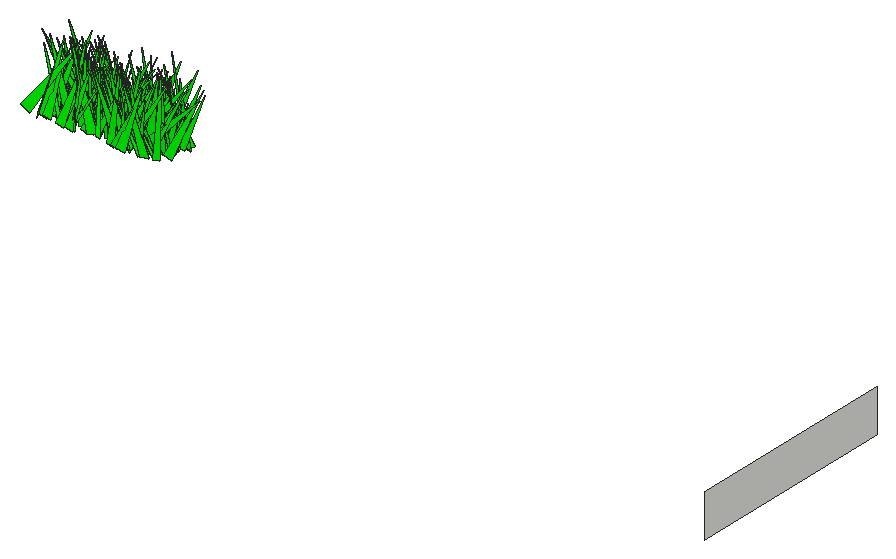
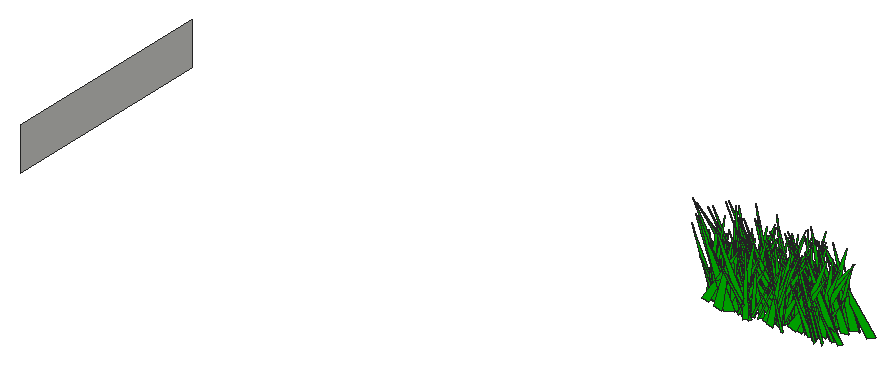
# SketchUp Ruby script. Lengths in inches.
U = 1.inch
M = Sketchup.active_model
def pt(a) = Geom::Point3d.new(a.map { |v| v * U })
def face(e, loops, mat)
  f = e.add_face(loops[0].map { |a| pt(a) })
  loops[1..].each { |l| e.add_face(l.map { |a| pt(a) }).erase! }
  f.material = f.back_material = mat if mat
  f
end
# faces: each face lists its corners as indices into pts; further lists are holes
def faces(e, pts, list, mat = nil) = list.each { |f| face(e, (f[0].is_a?(Array) ? f : [f]).map { |l| l.map { |i| pts[i] } }, mat) }
# xy, xz, yz: faces in a plane at the given z, y or x. An outline is a flat list of corners, or four numbers for a rectangle; further outlines are holes
def ring(l) = l.size == 4 ? [[l[0], l[1]], [l[2], l[1]], [l[2], l[3]], [l[0], l[3]]] : l.each_slice(2).to_a
def flat(e, list, mat, &to3) = list.each { |f| face(e, (f[0].is_a?(Array) ? f : [f]).map { |l| ring(l).map { |u, v| to3.(u, v) } }, mat) }
def xy(e, z, list, mat = nil) = flat(e, list, mat) { |x, y| [x, y, z] }
def xz(e, y, list, mat = nil) = flat(e, list, mat) { |x, z| [x, y, z] }
def yz(e, x, list, mat = nil) = flat(e, list, mat) { |y, z| [x, y, z] }
def lines(e, pts, list) = list.each { |a, b| e.add_line(pt(pts[a]), pt(pts[b])) }
# prism: a flat outline (further loops are holes) pulled along v
def prism(e, loops, v, mat = nil)
  f = face(e, loops, mat); d = Geom::Vector3d.new(v.map { |x| x * U })
  f.pushpull(f.normal.samedirection?(d) ? d.length : -d.length)
end
def box(e, o, s, mat = nil) = prism(e, [[o, [o[0] + s[0], o[1], o[2]], [o[0] + s[0], o[1] + s[1], o[2]], [o[0], o[1] + s[1], o[2]]]], [0, 0, s[2]], mat)
def at(x, y, z, deg = 0) = Geom::Transformation.translation(pt([x, y, z])) * Geom::Transformation.rotation(ORIGIN, Z_AXIS, deg.degrees)
def axes(o, x, y, z) = Geom::Transformation.new([*x, 0, *y, 0, *z, 0, *pt(o).to_a, 1])
def part(name) = M.definitions.add(name)
# library, detail: a bought-in or finely detailed component or shape, given as its bounding box
def library(name, o, s) = part(name).tap { |d| box(d.entities, o, s) }
def detail(e, o, s) = box(e.add_group.entities, o, s)
def put(e, d, t, mat = nil) = e.add_instance(d, t).tap { |i| i.material = mat if mat }
def group(e, t, mat = nil) = e.add_group.tap { |g| g.transformation = t; g.material = mat if mat }.entities
root = M.entities
M.materials.add("[0065_Lime]").color = [0, 255, 0]
c1 = part("fur_instance\#9")
p = [[0.8125,0,1.79],[0.67,-0.02,1.48],[0,-0.11,0],[0,0.11,0]]
faces(c1.entities,p,[[0,1,2,3]])
yz(root,282.96,[[0,-11.8125,39.75,-3.9375]])
put(root,c1,axes([141.5625,19.58,1.48],[2.20654,1.20218,2.33914],[-8.01635,0.06988,3.7999],[4.14751,-0.50452,6.10002]),"[0065_Lime]")
put(root,c1,axes([147.93,19.65,1.48],[-6.97873,0.43873,0.69681],[-2.96337,-0.98079,1.05602],[1.30411,0.11912,6.1285]),"[0065_Lime]")
put(root,c1,axes([144.33,18.92,1.48],[7.25336,-0.09629,0.71181],[0.1838,0.90456,2.86128],[-1.09619,-0.48551,5.18975]),"[0065_Lime]")
put(root,c1,axes([143.88,23.88,1.48],[1.3632,-0.63069,1.12453],[4.15726,0.06795,-2.05747],[2.18484,0.26422,3.21328]),"[0065_Lime]")
put(root,c1,axes([144.875,19.43,1.48],[-3.49359,1.08943,2.25762],[-7.42243,-0.60007,2.10352],[3.56638,-0.18169,6.58944]),"[0065_Lime]")
put(root,c1,axes([150.37,22.14,1.48],[-2.75165,-1.05841,0.96268],[7.17807,-0.29998,2.52342],[-2.57099,0.29525,6.01494]),"[0065_Lime]")
put(root,c1,axes([145.71,19.36,1.48],[-0.65738,0.93907,0.42813],[-6.48617,-0.10788,1.33939],[1.6937,-0.04864,5.29548]),"[0065_Lime]")
put(root,c1,axes([148.99,20.83,1.48],[-4.18903,-0.24167,0.3067],[1.732,-0.54103,1.36687],[-0.31652,0.23788,3.4204]),"[0065_Lime]")
put(root,c1,axes([145.5,20.31,1.48],[7.3444,0.3612,0.82059],[-2.31076,1.02444,-1.4263],[-1.5118,0.18888,6.16656]),"[0065_Lime]")
put(root,c1,axes([147.78,23.43,1.48],[3.54324,-1.13333,0.24164],[7.72696,0.48952,1.96765],[-2.33086,-0.10005,6.89022]),"[0065_Lime]")
put(root,c1,axes([147.25,20.59,1.48],[4.55951,-0.27108,1.43916],[1.50494,0.68003,1.13749],[-2.14174,-0.09925,3.86308]),"[0065_Lime]")
put(root,c1,axes([149.5,23.12,1.48],[-2.25393,-1.02556,0.82554],[7.20883,-0.276,1.53316],[-1.52654,0.21089,6.02119]),"[0065_Lime]")
put(root,c1,axes([147.41,21.64,1.48],[-3.74761,0.46815,0.23905],[-2.94612,-0.49143,1.69066],[1.58322,0.19368,3.71191]),"[0065_Lime]")
put(root,c1,axes([146.61,20.24,1.48],[-2.35602,0.71684,1.55449],[-5.12228,-0.39111,0.90693],[1.85452,-0.16956,4.47986]),"[0065_Lime]")
put(root,c1,axes([146.07,25.37,1.48],[6.49206,0.06434,1.15893],[-0.05568,0.90105,-1.46982],[-1.49551,0.24575,5.08571]),"[0065_Lime]")
put(root,c1,axes([144.83,23.57,1.48],[3.73059,0.98054,1.41858],[-7.08226,0.45258,1.8405],[1.25541,-0.36059,6.1675]),"[0065_Lime]")
put(root,c1,axes([145,23.73,1.48],[2.36799,1.27418,0.18786],[-8.9088,0.32039,1.48209],[1.70623,-0.09551,7.47774]),"[0065_Lime]")
put(root,c1,axes([152.77,21.72,1.48],[-6.46009,0.95745,0.30947],[-6.30621,-0.80939,-3.18772],[-2.6084,-0.41445,6.94037]),"[0065_Lime]")
put(root,c1,axes([149.78,19.83,1.48],[-2.56954,1.1411,1.85865],[-8.37179,-0.30358,-1.41229],[-1.03904,-0.3759,6.78277]),"[0065_Lime]")
put(root,c1,axes([145.34,23.82,1.48],[6.35731,-0.22767,0.53306],[1.74475,0.84708,-1.6442],[-0.10245,0.29824,5.07681]),"[0065_Lime]")
put(root,c1,axes([145.48,20.91,1.48],[5.10197,0.98969,1.68963],[-7.32568,0.66151,1.65177],[0.5059,-0.40195,6.87867]),"[0065_Lime]")
put(root,c1,axes([148.52,22.64,1.48],[-4.37999,-0.37273,0.87769],[2.35536,-0.6265,-1.13841],[1.62873,-0.09636,4.00656]),"[0065_Lime]")
put(root,c1,axes([148.85,24.07,1.48],[-4.93438,-0.47308,0.40197],[3.03876,-0.66768,-1.65014],[1.53121,-0.19947,4.57013]),"[0065_Lime]")
put(root,c1,axes([147.08,22.4,1.48],[6.97665,0.36677,2.16628],[-3.21314,0.99415,1.20661],[-1.89239,-0.33583,5.93769]),"[0065_Lime]")
put(root,c1,axes([147.11,25.87,1.48],[5.53718,0.0797,0.9196],[-0.81995,0.76935,1.03237],[-0.96306,-0.1968,4.40831]),"[0065_Lime]")
put(root,c1,axes([150.49,21.42,1.48],[-4.93557,-0.23453,0.41154],[1.74339,-0.66937,1.05115],[0.04838,0.19489,4.10557]),"[0065_Lime]")
put(root,c1,axes([151.4,24.46,1.48],[-5.52806,-1.01005,1.40888],[7.36884,-0.72767,1.64938],[-0.60725,0.36488,7.18923]),"[0065_Lime]")
put(root,c1,axes([148.9,23.33,1.48],[-4.95765,-0.84883,1.39379],[5.90771,-0.7345,-1.08569],[2.12734,0.06158,6.26314]),"[0065_Lime]")
put(root,c1,axes([147.18,22.61,1.48],[5.87849,0.29778,0.30468],[-1.98317,0.80905,-1.17995],[-0.83558,0.17474,4.944]),"[0065_Lime]")
put(root,c1,axes([148.66,22.27,1.48],[-3.00842,-0.53467,0.10404],[3.43756,-0.39133,-1.62121],[1.63632,-0.16091,3.59711]),"[0065_Lime]")
put(root,c1,axes([151.14,21.84,1.48],[-3.35195,0.85295,0.90617],[-6.1043,-0.43203,-1.31319],[-0.90765,-0.24434,5.48523]),"[0065_Lime]")
put(root,c1,axes([152.37,24.53,1.48],[-3.97671,0.93782,0.27867],[-6.39186,-0.51742,-2.00237],[-1.95047,-0.21646,5.99377]),"[0065_Lime]")
put(root,c1,axes([151.22,23.7,1.48],[-1.49671,0.82532,1.20922],[-5.79693,-0.13252,-1.71648],[-1.76135,-0.26515,4.62172]),"[0065_Lime]")
put(root,c1,axes([147.38,23.35,1.48],[1.15932,-0.85561,0.4723],[5.95948,0.1393,-1.22246],[1.37745,0.11743,4.89139]),"[0065_Lime]")
put(root,c1,axes([147.58,20.61,1.48],[1.71149,0.52944,0.12124],[-3.59338,0.22204,1.07239],[1.14269,-0.09474,3.19072]),"[0065_Lime]")
put(root,c1,axes([150.46,22.47,1.48],[1.53529,0.56905,0.27796],[-3.6294,0.21508,-1.49067],[-1.82868,0.05089,3.19191]),"[0065_Lime]")
put(root,c1,axes([149.52,23.63,1.48],[-4.03165,0.0597,1.8592],[-1.0991,-0.6155,-0.91462],[2.04862,-0.21273,3.16818]),"[0065_Lime]")
put(root,c1,axes([149.93,22.65,1.48],[-5.98029,-0.8429,0.18918],[5.44661,-0.78127,-2.72487],[2.52406,-0.31121,6.32814]),"[0065_Lime]")
put(root,c1,axes([147.69,25.28,1.48],[8.61099,-0.37367,0.75747],[2.45007,1.20083,1.42172],[-1.39136,-0.19804,7.19149]),"[0065_Lime]")
put(root,c1,axes([148.4375,24.65,1.48],[-0.04705,-1.17072,0.26335],[8.10686,-0.01706,-1.58237],[1.94856,0.04269,6.58971]),"[0065_Lime]")
put(root,c1,axes([149.85,22.76,1.48],[-6.12929,-0.74533,0.16535],[4.24135,-0.71392,-3.81017],[3.19162,-0.48262,5.38089]),"[0065_Lime]")
put(root,c1,axes([153.17,24.05,1.48],[-3.64838,-0.56917,0.80639],[3.93076,-0.40758,2.12677],[-1.39242,0.34074,3.89092]),"[0065_Lime]")
put(root,c1,axes([152.62,23.41,1.48],[-1.12028,1.15408,0.64786],[-8.03924,-0.12719,-1.60528],[-1.85986,-0.14535,6.54857]),"[0065_Lime]")
put(root,c1,axes([148.71,24.83,1.48],[2.84326,0.64249,0.39365],[-4.54228,0.38012,0.91821],[0.71259,-0.14057,4.28228]),"[0065_Lime]")
put(root,c1,axes([148.64,18.74,1.48],[2.22567,0.92219,0.99487],[-6.58515,0.27352,1.25154],[1.09663,-0.22921,5.49624]),"[0065_Lime]")
put(root,c1,axes([151.48,21.18,1.48],[-8.34339,-0.0857,2.24479],[-0.02277,-1.20659,-1.59957],[2.82621,-0.26272,6.61406]),"[0065_Lime]")
put(root,c1,axes([149.93,24.47,1.48],[4.72063,0.10631,0.85352],[-0.3936,0.64949,-1.27031],[-1.23225,0.19979,3.67549]),"[0065_Lime]")
put(root,c1,axes([151.53,23.91,1.48],[-4.16121,-0.53442,0.1089],[3.60478,-0.56246,-1.35649],[1.21978,-0.1609,4.38028]),"[0065_Lime]")
put(root,c1,axes([153.41,20.67,1.48],[3.38639,-0.8607,4.01971],[6.71512,0.71024,1.35296],[-4.10446,0.45187,5.52997]),"[0065_Lime]")
put(root,c1,axes([149.8,19.63,1.48],[8.32669,-0.46304,2.49552],[3.88184,1.1975,-1.12428],[-2.28087,0.34763,7.19685]),"[0065_Lime]")
put(root,c1,axes([152.74,20.86,1.48],[-7.78088,-0.56548,0.89942],[3.74968,-1.09155,-1.53398],[1.83234,-0.16754,6.9584]),"[0065_Lime]")
put(root,c1,axes([151.46,18.67,1.48],[7.41008,0.10379,2.59282],[0.16748,1.09537,-1.78601],[-3.26775,0.2915,5.78804]),"[0065_Lime]")
put(root,c1,axes([151.44,20.45,1.48],[5.13469,0.907,1.4446],[-6.32228,0.7604,-1.12939],[-2.20133,-0.06827,6.61322]),"[0065_Lime]")
put(root,c1,axes([147.3,20.35,1.48],[7.19198,-0.75486,0.91121],[5.17085,0.84533,-3.53719],[1.83736,0.57576,6.38791]),"[0065_Lime]")
put(root,c1,axes([153.84,19.66,1.48],[4.02373,-1.03653,3.45136],[7.56263,0.73794,1.59281],[-3.90173,0.3614,6.64659]),"[0065_Lime]")
put(root,c1,axes([151.38,24.125,1.48],[-2.16031,-0.73135,0.90472],[5.04667,-0.33506,-1.10284],[1.69026,0.06566,4.44911]),"[0065_Lime]")
put(root,c1,axes([150.92,19.02,1.48],[7.24147,-0.41945,0.98876],[2.5105,0.9975,2.01423],[-2.0212,-0.26379,6.04433]),"[0065_Lime]")
put(root,c1,axes([148.58,20.76,1.48],[9.08947,-0.29649,0.75138],[2.29764,1.20426,-2.46681],[-0.16186,0.44489,7.17804]),"[0065_Lime]")
put(root,c1,axes([154.72,22.74,1.48],[-3.76527,-0.75846,0.57438],[5.33693,-0.49057,1.44123],[-1.07245,0.22164,5.15554]),"[0065_Lime]")
put(root,c1,axes([154.72,24.29,1.48],[-2.54464,-0.7055,0.33945],[4.83651,-0.32369,1.44572],[-1.4107,0.16285,4.34427]),"[0065_Lime]")
put(root,c1,axes([150.35,18.71,1.48],[4.38909,0.9203,1.169],[-6.69443,0.58778,1.12437],[0.37952,-0.27507,6.31365]),"[0065_Lime]")
put(root,c1,axes([153.94,20.47,1.48],[-0.96663,0.63537,1.6368],[-4.81677,-0.05457,-1.17223],[-1.13723,-0.30891,3.57374]),"[0065_Lime]")
put(root,c1,axes([154.33,23.8,1.48],[-7.59822,-0.28511,1.78301],[2.59248,-1.04765,1.69604],[1.48355,0.37049,6.16814]),"[0065_Lime]")
put(root,c1,axes([154.48,23.97,1.48],[-2.53235,-0.52716,0.87742],[3.7837,-0.28706,1.44605],[-0.95974,0.25921,3.38582]),"[0065_Lime]")
put(root,c1,axes([156.46,25.23,1.48],[-7.88996,0.41333,1.22187],[-3.29694,-0.95302,-3.28318],[-0.19697,-0.60454,6.01111]),"[0065_Lime]")
put(root,c1,axes([155.04,21.24,1.48],[-1.43811,-0.78387,1.02946],[5.51855,-0.14186,1.48107],[-1.50546,0.22877,4.44572]),"[0065_Lime]")
put(root,c1,axes([155.22,25.23,1.48],[-7.20987,0.33169,0.69678],[-2.22794,-1.01378,0.91794],[1.1584,0.11463,6.10225]),"[0065_Lime]")
put(root,c1,axes([156.16,25.41,1.48],[-0.2011,1.02006,3.52858],[-7.88493,0.19778,-2.2132],[-3.05677,-0.57728,5.47681]),"[0065_Lime]")
put(root,c1,axes([154.23,25.31,1.48],[-4.35759,-0.46082,1.86211],[3.86103,-0.60878,0.92987],[1.04299,0.32833,4.33759]),"[0065_Lime]")
put(root,c1,axes([155.28,25.25,1.48],[-8.00806,-0.35289,0.85298],[2.22102,-1.11207,-1.62064],[1.57282,-0.22638,6.63151]),"[0065_Lime]")
put(root,c1,axes([153.45,20.19,1.48],[-7.20917,-0.72621,1.79727],[4.56066,-1.05093,-2.12551],[3.28507,-0.13467,6.895]),"[0065_Lime]")
put(root,c1,axes([154.09,24.29,1.48],[-5.70536,0.11358,1.45263],[-0.1549,-0.79599,1.683],[1.95413,0.26852,4.37458]),"[0065_Lime]")
put(root,c1,axes([152.62,21.0625,1.48],[4.29648,-0.33876,0.25657],[2.25304,0.58855,1.07665],[-0.91399,-0.14164,3.86006]),"[0065_Lime]")
put(root,c1,axes([150.33,19.49,1.48],[7.27024,0.26556,0.0507],[-1.86508,1.00136,1.19848],[0.31155,-0.20255,5.99156]),"[0065_Lime]")
put(root,c1,axes([151.98,20.91,1.48],[-2.55544,1.00319,3.00371],[-7.47975,-0.49613,1.34209],[2.94249,-0.38993,6.02017]),"[0065_Lime]")
put(root,c1,axes([152.3,19.62,1.48],[0.28077,0.58795,0.75334],[-4.03898,-0.00728,1.18646],[1.43229,-0.13579,3.1981]),"[0065_Lime]")
put(root,c1,axes([155.33,24.73,1.48],[-3.58078,0.71828,2.38822],[-5.89485,-0.43801,-1.43354],[0.02077,-0.48118,4.86998]),"[0065_Lime]")
put(root,c1,axes([151.82,22.16,1.48],[3.01702,-0.90611,0.28276],[6.33306,0.40461,-1.26182],[1.26299,0.13567,5.65178]),"[0065_Lime]")
put(root,c1,axes([151.69,21.15,1.48],[8.39239,-0.20933,0.53718],[1.31319,1.15707,1.5344],[-0.96479,-0.24595,6.76127]),"[0065_Lime]")
put(root,c1,axes([156.35,20.75,1.48],[-7.52113,-0.71578,0.28063],[4.96108,-1.04499,-1.34075],[1.20589,-0.16518,7.2662]),"[0065_Lime]")
put(root,c1,axes([157.73,21.33,1.48],[-1.94785,-1.28804,0.64989],[8.74484,-0.22346,2.50109],[-2.86169,0.19387,7.20056]),"[0065_Lime]")
put(root,c1,axes([155.39,21.25,1.48],[-7.42832,-0.4771,2.88553],[4.3499,-1.05876,1.54307],[2.27835,0.46588,6.46187]),"[0065_Lime]")
put(root,c1,axes([156.11,23.72,1.48],[1.781,1.05304,2.56561],[-7.67529,0.36746,-1.52867],[-2.68301,-0.35219,6.07616]),"[0065_Lime]")
put(root,c1,axes([156.88,20.89,1.48],[1.90523,1.03845,0.88855],[-6.56005,0.30835,-2.76903],[-3.5741,-0.0124,5.55605]),"[0065_Lime]")
put(root,c1,axes([155.4,25.85,1.48],[4.84781,-0.71048,1.80407],[4.45556,0.74835,1.95395],[-3.26066,-0.03372,5.35221]),"[0065_Lime]")
put(root,c1,axes([155.5,24.87,1.48],[-6.01251,-0.07951,1.18868],[-0.07482,-0.79869,-2.04062],[1.56529,-0.34359,4.46836]),"[0065_Lime]")
put(root,c1,axes([155.09,19.93,1.48],[-3.12346,-0.37436,0.06154],[2.53893,-0.42291,-0.9469],[0.81078,-0.11786,3.20227]),"[0065_Lime]")
put(root,c1,axes([152.89,26.2,1.48],[7.59512,-0.18655,1.04839],[1.1104,1.07159,1.06708],[-1.48014,-0.15337,6.1802]),"[0065_Lime]")
put(root,c1,axes([155.14,19.45,1.48],[6.226,-0.22227,2.88785],[2.65362,0.93142,-1.38304],[-2.83988,0.38304,5.03884]),"[0065_Lime]")
put(root,c1,axes([153.76,23.42,1.48],[-5.28443,-0.93143,0.4422],[5.31678,-0.65024,-3.85639],[3.99567,-0.36662,5.71627]),"[0065_Lime]")
put(root,c1,axes([156.02,24.8,1.48],[-5.1908,0.03711,1.21944],[0.32478,-0.70436,1.63291],[1.48719,0.28334,3.89964]),"[0065_Lime]")
put(root,c1,axes([156.3125,21.1,1.48],[2.52612,-0.69593,1.29459],[4.65487,0.41339,1.43681],[-2.32242,0.07159,4.28797]),"[0065_Lime]")
put(root,c1,axes([158.68,22.91,1.48],[-2.68251,1.17397,1.04334],[-8.11576,-0.30489,-2.31033],[-2.36204,-0.28568,6.7532]),"[0065_Lime]")
put(root,c1,axes([156.9,22.63,1.48],[-5.16673,0.15232,0.28892],[-0.83796,-0.66391,1.81356],[0.77393,0.29802,3.89243]),"[0065_Lime]")
put(root,c1,axes([159.56,21.79,1.48],[-4.72379,-0.97799,0.10368],[6.59306,-0.62163,2.26177],[-2.23342,0.23343,6.45744]),"[0065_Lime]")
put(root,c1,axes([156.28,19.99,1.48],[-4.01172,-0.29727,1.90189],[2.93231,-0.54719,1.22651],[1.15925,0.3554,3.47924]),"[0065_Lime]")
put(root,c1,axes([156.68,23.03,1.48],[-5.76365,0.40626,0.41076],[-2.48098,-0.75796,2.08694],[1.56801,0.29405,4.81194]),"[0065_Lime]")
put(root,c1,axes([156.21,21.74,1.48],[-4.37641,0.43472,0.42348],[-2.7508,-0.59211,1.55872],[1.50838,0.18148,4.07128]),"[0065_Lime]")
put(root,c1,axes([158.01,25.23,1.48],[-6.5955,-0.24617,0.26109],[1.6658,-0.91386,-1.02963],[0.63015,-0.16072,5.45456]),"[0065_Lime]")
put(root,c1,axes([154.59,20.5,1.48],[7.92793,-0.30745,2.46575],[3.1632,1.08396,-2.20015],[-1.99265,0.49749,6.31762]),"[0065_Lime]")
put(root,c1,axes([158.76,20.57,1.48],[-9.25784,-0.04517,1.02604],[-0.05316,-1.25881,-2.17449],[1.30063,-0.37299,7.2144]),"[0065_Lime]")
put(root,c1,axes([155.42,23.04,1.48],[-2.36096,-0.92147,1.78698],[6.63284,-0.39406,-1.0109],[1.95828,0.22377,5.57842]),"[0065_Lime]")
put(root,c1,axes([156.72,23.74,1.48],[2.78258,0.70896,0.00093],[-4.78444,0.37084,-1.4871],[-1.60142,0.12393,4.44452]),"[0065_Lime]")
put(root,c1,axes([155.57,22.92,1.48],[5.07132,0.6691,2.39223],[-5.52794,0.686,1.32418],[-0.87465,-0.45608,5.50134]),"[0065_Lime]")
put(root,c1,axes([159.18,19.16,1.48],[-0.52294,-1.097,1.19832],[7.61737,-0.01031,1.88328],[-2.25665,0.21942,6.07938]),"[0065_Lime]")
put(root,c1,axes([159.01,25.46,1.48],[-5.35719,0.09003,0.06746],[-0.60833,-0.73573,0.939],[0.21754,0.15973,4.28703]),"[0065_Lime]")
put(root,c1,axes([157.11,22.54,1.48],[-3.10367,0.50614,0.36796],[-3.37079,-0.43284,1.13904],[1.34781,0.083,3.69598]),"[0065_Lime]")
put(root,c1,axes([156.17,22.32,1.48],[-5.60706,0.5759,1.97802],[-3.02373,-0.83775,2.50214],[3.68344,0.18895,5.06502]),"[0065_Lime]")
put(root,c1,axes([159.9,23.18,1.48],[-3.14727,-0.80554,0.97244],[5.64426,-0.36646,1.91441],[-1.56048,0.29918,4.96313]),"[0065_Lime]")
put(root,c1,axes([159.6,20.27,1.48],[-2.19282,0.9655,0.9674],[-6.78686,-0.25528,-1.64132],[-1.6011,-0.24022,5.6324]),"[0065_Lime]")
put(root,c1,axes([154.58,19.76,1.48],[5.93857,0.64917,0.95509],[-4.73808,0.77502,1.84028],[0.52212,-0.35058,5.83684]),"[0065_Lime]")
put(root,c1,axes([158.75,21.01,1.48],[0.66312,-0.58857,1.20212],[4.13954,0.15801,1.0815],[-1.61013,0.16383,3.27555]),"[0065_Lime]")
put(root,c1,axes([159.34,20.43,1.48],[-0.31563,1.06536,1.63002],[-7.65947,0.01857,-1.38808],[-1.68224,-0.28445,6.01427]),"[0065_Lime]")
put(root,c1,axes([153.99,24.07,1.48],[2.643,-1.23625,0.72196],[8.31345,0.30305,-2.74766],[3.0127,0.24828,6.94871]),"[0065_Lime]")
put(root,c1,axes([153.91,23.78,1.48],[3.0131,1.08274,1.05681],[-7.15543,0.30368,3.07255],[3.1401,-0.34695,5.98745]),"[0065_Lime]")
put(root,c1,axes([155.99,23.86,1.48],[4.35296,-0.63543,0.66091],[4.58173,0.58865,-1.00171],[0.3421,0.20167,5.00634]),"[0065_Lime]")
put(root,c1,axes([157.5,24.84,1.48],[-0.3071,-0.74818,1.36568],[5.36471,-0.10495,-1.12854],[1.54547,0.21565,4.18881]),"[0065_Lime]")
put(root,c1,axes([157.97,18.77,1.48],[-4.12814,-0.96284,2.72016],[7.01912,-0.68859,-1.11942],[2.97765,0.28834,6.40993]),"[0065_Lime]")
put(root,c1,axes([159.0625,25.23,1.48],[4.73585,-0.39516,1.43229],[2.43057,0.70671,1.21616],[-2.25862,-0.06806,4.31196]),"[0065_Lime]")
put(root,c1,axes([153.98,24.17,1.48],[3.44387,1.03674,0.63109],[-6.23789,0.33961,3.82781],[4.01572,-0.36157,5.40478]),"[0065_Lime]")
put(root,c1,axes([154.625,21.77,1.48],[4.38225,1.102,0.39331],[-7.2405,0.53615,3.03905],[3.05174,-0.3104,6.64561]),"[0065_Lime]")
put(root,c1,axes([161.04,26.05,1.48],[-6.49027,-0.10385,0.70791],[0.46346,-0.8847,-1.5375],[1.04346,-0.25299,5.08608]),"[0065_Lime]")
put(root,c1,axes([161.21,23.3,1.48],[3.41777,-0.87909,3.36339],[6.66704,0.64852,1.19742],[-3.43315,0.38426,5.67367]),"[0065_Lime]")
put(root,c1,axes([162.05,24.43,1.48],[-2.58515,0.74033,0.19401],[-5.04051,-0.33584,-1.49515],[-1.55175,-0.14244,4.53343]),"[0065_Lime]")
put(root,c1,axes([159.38,26.52,1.48],[-6.57546,-0.71959,1.5329],[4.31958,-0.93979,-2.52334],[3.33421,-0.20158,6.29213]),"[0065_Lime]")
put(root,c1,axes([160.95,20.82,1.48],[-7.83976,-0.02554,1.8745],[-0.32041,-1.1219,-1.39893],[2.28933,-0.24449,6.22338]),"[0065_Lime]")
put(root,c1,axes([161.39,24.91,1.48],[3.23968,1.06743,2.07906],[-7.38621,0.54802,-1.81308],[-3.11173,-0.18949,6.4682]),"[0065_Lime]")
put(root,c1,axes([156.93,23.41,1.48],[9.20584,0.2249,0.83476],[-1.72408,1.28802,0.95212],[-0.80141,-0.18753,7.5406]),"[0065_Lime]")
put(root,c1,axes([164.16,22.32,1.48],[-6.6223,0.79591,0.65888],[-5.48517,-0.83355,-2.73647],[-1.62826,-0.42904,6.53871]),"[0065_Lime]")
put(root,c1,axes([159.83,22.7,1.48],[-3.06776,-0.66305,0.468],[4.44196,-0.43412,-1.34439],[1.69267,-0.06246,4.37618]),"[0065_Lime]")
put(root,c1,axes([160.64,19.91,1.48],[-5.3506,-0.65059,0.19616],[4.23819,-0.70735,-2.12452],[1.87953,-0.25709,5.34901]),"[0065_Lime]")
put(root,c1,axes([163.14,21.61,1.48],[-4.46745,0.93475,1.12691],[-6.68011,-0.56154,-1.91371],[-1.24375,-0.34154,6.23068]),"[0065_Lime]")
put(root,c1,axes([159.18,25.07,1.48],[4.53579,0.14608,0.45506],[-0.78736,0.60687,-1.33528],[-0.87961,0.21003,3.54179]),"[0065_Lime]")
put(root,c1,axes([162.58,25.39,1.48],[-2.95805,-0.8962,0.28003],[6.26525,-0.39677,1.23869],[-1.24172,0.13299,5.58287]),"[0065_Lime]")
put(root,c1,axes([159.76,18.89,1.48],[4.65771,-0.43668,0.43509],[2.77559,0.63136,1.57428],[-1.49659,-0.18811,4.27379]),"[0065_Lime]")
put(root,c1,axes([158.65,20.59,1.48],[8.12662,-0.36345,1.06489],[2.33966,1.14558,1.28809],[-1.7117,-0.1597,6.81639]),"[0065_Lime]")
put(root,c1,axes([161.51,18.69,1.48],[-4.26419,0.06926,0.68581],[-0.24826,-0.59012,0.97557],[0.94454,0.15755,3.35258]),"[0065_Lime]")
put(root,c1,axes([158.73,18.59,1.48],[1.9833,-0.67955,0.53103],[4.72582,0.24278,-1.26755],[1.21652,0.16475,4.05829]),"[0065_Lime]")
put(root,c1,axes([164.66,22.29,1.48],[-4.23474,-0.85648,0.26763],[5.5848,-0.52093,2.60532],[-2.46364,0.2913,5.44594]),"[0065_Lime]")
put(root,c1,axes([161.42,22.46,1.48],[5.38601,-0.5007,1.95194],[3.04661,0.82644,1.5415],[-3.02873,-0.05907,5.02175]),"[0065_Lime]")
put(root,c1,axes([163.14,19,1.48],[-5.99672,0.12271,0.68376],[-1.1454,-0.76872,-2.02378],[0.39654,-0.36479,4.49465]),"[0065_Lime]")
put(root,c1,axes([163.02,22.02,1.48],[-5.40537,-0.05138,0.59987],[-0.02009,-0.67989,-2.0713],[0.82291,-0.35412,3.88973]),"[0065_Lime]")
put(root,c1,axes([159.83,19.36,1.48],[7.72408,0.62598,2.15563],[-4.94888,1.08934,1.13279],[-1.54164,-0.36061,7.1639]),"[0065_Lime]")
put(root,c1,axes([160.01,20.22,1.48],[-0.87959,0.70997,2.42689],[-5.41768,-0.26108,1.2602],[2.25363,-0.35054,3.97672]),"[0065_Lime]")
put(root,c1,axes([159.35,24.23,1.48],[7.28029,0.41827,0.95398],[-3.15426,1.00692,1.13317],[-0.53536,-0.24458,6.29659]),"[0065_Lime]")
put(root,c1,axes([165.08,21.04,1.48],[-4.82595,0.74526,0.97783],[-5.27369,-0.58622,-2.24949],[-1.32754,-0.38046,5.3815]),"[0065_Lime]")
put(root,c1,axes([161.27,23.53,1.48],[7.38169,0.70032,0.10299],[-4.25214,0.90099,-3.65136],[-2.60275,0.51423,6.25735]),"[0065_Lime]")
put(root,c1,axes([160.04,18.54,1.48],[2.72011,-0.934,1.70483],[6.90009,0.31641,-1.47548],[0.98075,0.3643,5.65242]),"[0065_Lime]")
put(root,c1,axes([165.16,20.18,1.48],[-6.63342,-0.54894,0.64495],[3.96964,-0.88997,1.63113],[-0.36337,0.29867,6.04572]),"[0065_Lime]")
put(root,c1,axes([164.13,18.88,1.48],[-1.42131,-1.06315,1.08577],[7.54128,-0.15661,1.39291],[-1.46783,0.22481,6.10501]),"[0065_Lime]")
put(root,c1,axes([159.55,19.68,1.48],[5.90128,-0.68641,1.37741],[5.15699,0.75588,-1.99634],[0.36705,0.4158,5.90291]),"[0065_Lime]")
put(root,c1,axes([163.28,19.66,1.48],[2.89513,-0.96955,1.0871],[6.61505,0.44452,1.62871],[-2.37382,0.05627,5.86449]),"[0065_Lime]")
put(root,c1,axes([159.78,21.22,1.48],[6.13171,0.75858,1.25246],[-5.6133,0.82443,1.45063],[0.07141,-0.33092,6.48494]),"[0065_Lime]")
put(root,c1,axes([159.78,25.78,1.48],[1.98317,1.17608,1.17468],[-8.24277,0.21628,1.95157],[2.04752,-0.26844,6.71875]),"[0065_Lime]")
put(root,c1,axes([164.84,20.01,1.48],[-5.47734,0.21995,0.24529],[-1.58153,-0.73084,-1.40655],[-0.19953,-0.24505,4.41506]),"[0065_Lime]")
put(root,c1,axes([164.5,23.18,1.48],[-6.93567,-0.18296,1.12254],[1.62508,-0.95216,1.44297],[0.97928,0.28427,5.55579]),"[0065_Lime]")
put(root,c1,axes([158.67,26.26,1.48],[6.21547,0.55512,0.10644],[-3.61641,0.7848,2.57027],[1.59551,-0.3837,5.41114]),"[0065_Lime]")
put(root,c1,axes([161.56,22.21,1.48],[4.39773,-0.07996,0.5156],[0.33914,0.59403,1.17295],[-0.78139,-0.19219,3.41095]),"[0065_Lime]")
put(root,c1,axes([163.49,21.99,1.48],[5.55652,0.60164,0.70334],[-3.0079,0.66959,-3.47017],[-3.16734,0.41958,4.52936]),"[0065_Lime]")
put(root,c1,axes([160.875,19.18,1.48],[1.61517,0.64176,0.66364],[-4.36217,0.16874,1.55662],[1.5797,-0.19021,3.61991]),"[0065_Lime]")
put(root,c1,axes([160.39,23.28,1.48],[1.71289,0.9605,0.40679],[-6.44853,0.20132,2.03695],[2.32158,-0.14946,5.3578]),"[0065_Lime]")
put(root,c1,axes([162.71,25.19,1.48],[5.99014,-0.58456,0.5766],[3.62629,0.80148,2.3017],[-2.15832,-0.27576,5.46747]),"[0065_Lime]")
put(root,c1,axes([162.06,22.84,1.48],[3.49707,-0.51534,1.18166],[3.94285,0.46497,-0.9255],[-0.1203,0.25874,4.01673]),"[0065_Lime]")
put(root,c1,axes([164.52,26.45,1.48],[4.43289,-0.91757,1.31733],[5.91012,0.66132,2.27674],[-3.21454,-0.04947,6.00253]),"[0065_Lime]")
put(root,c1,axes([161.4375,20.58,1.48],[3.90421,-0.46781,0.99168],[3.49945,0.46758,-1.72433],[0.56897,0.3342,3.80069]),"[0065_Lime]")
put(root,c1,axes([164.55,24.02,1.48],[2.13725,-0.95279,1.47385],[6.7544,0.35155,1.13482],[-1.90725,0.17729,5.67047]),"[0065_Lime]")
put(root,c1,axes([162.9,19.07,1.48],[-3.77494,-0.67954,1.54904],[4.47911,-0.59311,-1.49656],[2.63644,0.03466,4.7605]),"[0065_Lime]")
put(root,c1,axes([166.06,23.67,1.48],[-3.25789,0.62477,1.54009],[-4.7427,-0.35177,-1.85614],[-0.92756,-0.39574,4.08131]),"[0065_Lime]")
put(root,c1,axes([167.45,25.71,1.48],[-4.90514,0.79609,0.0756],[-5.49527,-0.66417,-1.54904],[-1.381,-0.18472,5.89544]),"[0065_Lime]")
put(root,c1,axes([163.01,23.83,1.48],[3.92623,-0.10455,0.58086],[0.93974,0.52538,-1.03421],[-0.42468,0.19603,3.08157]),"[0065_Lime]")
put(root,c1,axes([160.37,19.46,1.48],[5.57351,-1.02741,0.75869],[7.13615,0.71101,-2.42194],[1.84515,0.35356,7.07519]),"[0065_Lime]")
put(root,c1,axes([164.72,22.42,1.48],[7.26549,-0.29502,2.66084],[1.39475,1.1074,1.59451],[-3.62814,-0.16507,5.9414]),"[0065_Lime]")
put(root,c1,axes([164.22,21.71,1.48],[3.65206,0.51163,0.18504],[-3.36426,0.48982,-1.44986],[-1.41086,0.15637,3.93624]),"[0065_Lime]")
put(root,c1,axes([161.29,20.22,1.48],[9.3538,-0.05371,0.56059],[0.48809,1.30046,-1.21351],[-0.61873,0.21393,7.51754]),"[0065_Lime]")
put(root,c1,axes([165.7,24.53,1.48],[-0.12334,0.90733,0.6911],[-6.4117,0.00403,-0.9344],[-1.14246,-0.12057,5.16942]),"[0065_Lime]")
put(root,c1,axes([160.11,23.09,1.48],[7.34756,-0.77769,1.08634],[5.41372,0.85952,-3.6082],[1.76231,0.60201,6.55492]),"[0065_Lime]")
put(root,c1,axes([164.74,23.3,1.48],[2.91461,0.71319,0.20368],[-4.90351,0.40536,-1.13625],[-1.33356,0.06821,4.62314]),"[0065_Lime]")
put(root,c1,axes([161.65,21.82,1.48],[3.84504,0.65451,0.18798],[-4.34584,0.48759,1.92598],[1.69199,-0.235,4.51966]),"[0065_Lime]")
put(root,c1,axes([163.57,20.5625,1.48],[-1.79976,-1.26289,0.61534],[8.73971,-0.27097,-1.72235],[2.2278,0.04279,7.25394]),"[0065_Lime]")
put(root,c1,axes([165.0625,25.38,1.48],[4.95131,-0.28631,1.50297],[1.39027,0.72183,1.5774],[-2.37338,-0.17448,4.05946]),"[0065_Lime]")
put(root,c1,axes([163.09,22.25,1.48],[3.8615,-0.54294,1.10962],[4.07652,0.48235,-1.47766],[0.41497,0.31386,4.19049]),"[0065_Lime]")
put(root,c1,axes([165.74,21.68,1.48],[-5.87952,0.0417,1.84515],[-1.0776,-0.82588,-1.64654],[2.01804,-0.31953,4.49658]),"[0065_Lime]")
put(root,c1,axes([165.72,24.76,1.48],[-6.08379,-0.52248,1.3701],[3.46969,-0.88568,-1.12384],[2.15031,-0.04913,5.68976]),"[0065_Lime]")
put(root,c1,axes([166.7,25.05,1.48],[-0.48923,0.65031,0.9174],[-4.57532,-0.01982,-1.14343],[-1.32537,-0.17161,3.60861]),"[0065_Lime]")
put(root,c1,axes([166.46,22.39,1.48],[-5.10144,0.21583,0.51015],[-1.2822,-0.69373,1.35122],[1.05282,0.20092,4.11753]),"[0065_Lime]")
put(root,c1,axes([167.06,24.86,1.48],[-8.27535,-0.47362,2.47832],[3.98231,-1.18435,1.21375],[2.18743,0.36439,7.16614]),"[0065_Lime]")
put(root,c1,axes([165.36,21.28,1.48],[-2.9662,-0.93636,1.19637],[6.59682,-0.45112,-1.00968],[1.74624,0.1137,5.84649]),"[0065_Lime]")
put(root,c1,axes([162.69,26.11,1.48],[2.26038,-1.2684,0.31432],[8.69639,0.29026,-2.1281],[2.45001,0.13993,7.26378]),"[0065_Lime]")
put(root,c1,axes([166.77,23.72,1.48],[-6.91809,-0.01749,1.83787],[-0.58167,-0.97319,-1.75893],[2.18684,-0.31417,5.34626]),"[0065_Lime]")
put(root,c1,axes([165.99,19.34,1.48],[5.88679,0.99938,0.92693],[-6.71197,0.83616,-2.00495],[-2.61344,0.10365,7.23713]),"[0065_Lime]")
put(root,c1,axes([167.41,21.19,1.48],[-4.80897,-0.33431,1.55603],[2.93011,-0.64622,1.33922],[0.8568,0.33359,4.15364]),"[0065_Lime]")
put(root,c1,axes([162.93,20.77,1.48],[4.08533,1.10715,0.3189],[-7.51353,0.52717,2.35684],[2.40418,-0.23382,6.82367]),"[0065_Lime]")
put(root,c1,axes([165.38,22.28,1.48],[0.77938,-0.82532,0.9184],[5.78546,0.06346,-1.33748],[1.51663,0.18204,4.63008]),"[0065_Lime]")
put(root,c1,axes([167.41,24.7,1.48],[2.0428,0.49518,0.45863],[-3.33242,0.29734,-0.93696],[-1.27728,0.0162,3.17802]),"[0065_Lime]")
put(root,c1,axes([167.4375,24.72,1.48],[-4.741,-0.93554,0.30242],[6.42337,-0.65795,-1.57697],[1.79037,-0.11684,6.45859]),"[0065_Lime]")
put(root,c1,axes([165.37,24.86,1.48],[4.0727,-0.24068,0.24561],[1.72495,0.54514,-1.02437],[0.22257,0.17927,3.44476]),"[0065_Lime]")
put(root,c1,axes([164.35,20.14,1.48],[6.52451,0.71268,0.41355],[-5.08255,0.9008,1.03628],[0.38677,-0.18493,6.64164]),"[0065_Lime]")
put(root,c1,axes([162.03,20.27,1.48],[6.47724,-0.94441,0.42098],[5.87646,0.7417,-4.06701],[3.3024,0.53251,6.41133]),"[0065_Lime]")
put(root,c1,axes([167.16,22.68,1.48],[6.07546,-0.086,1.05286],[0.21694,0.83907,1.46826],[-1.41523,-0.24056,4.74489]),"[0065_Lime]")
put(root,c1,axes([165.96,23.14,1.48],[3.08024,1.08251,0.48635],[-7.60985,0.40931,1.36055],[1.3397,-0.1639,6.61006]),"[0065_Lime]")
put(root,c1,axes([166.71,24.23,1.48],[4.88243,-0.72515,0.53898],[5.18734,0.66858,-0.94898],[0.40194,0.17987,5.70017]),"[0065_Lime]")
put(root,c1,axes([166.85,21.1,1.48],[4.83988,1.03943,0.64137],[-7.32818,0.64345,1.6456],[1.27938,-0.24652,6.99956]),"[0065_Lime]")
